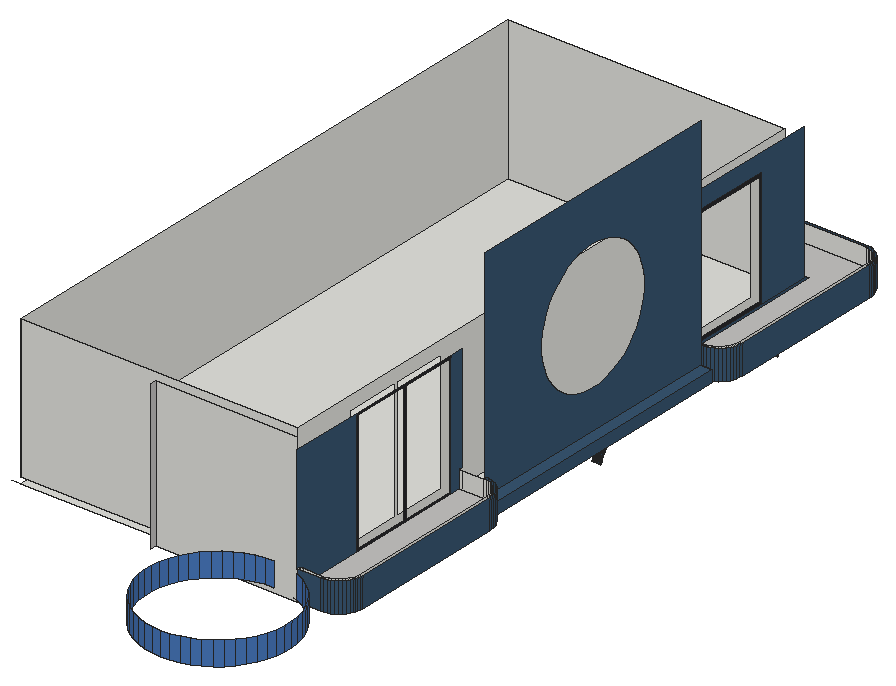
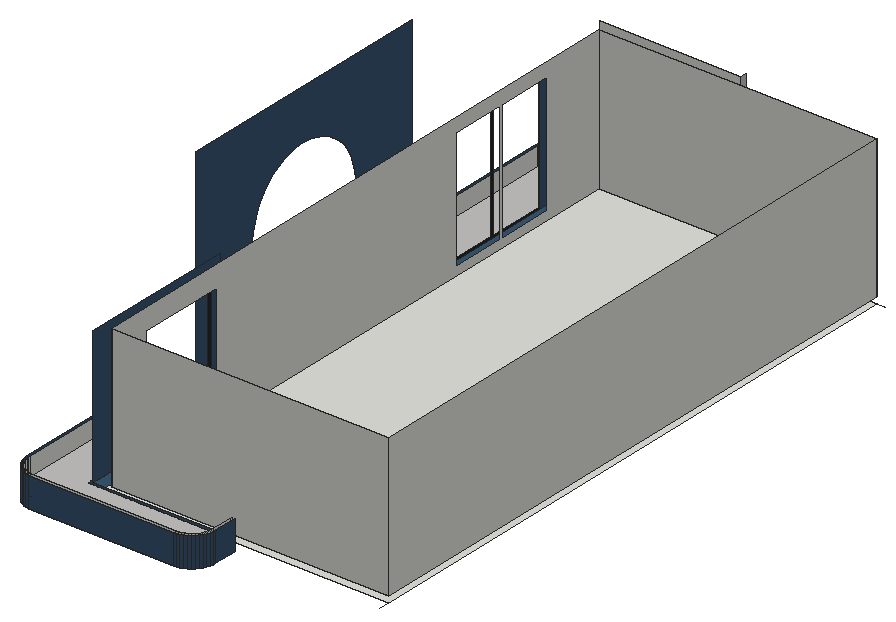
# SketchUp Ruby script. Lengths in inches.
U = 1.inch
M = Sketchup.active_model
def pt(a) = Geom::Point3d.new(a.map { |v| v * U })
def face(e, loops, mat)
  f = e.add_face(loops[0].map { |a| pt(a) })
  loops[1..].each { |l| e.add_face(l.map { |a| pt(a) }).erase! }
  f.material = f.back_material = mat if mat
  f
end
# faces: each face lists its corners as indices into pts; further lists are holes
def faces(e, pts, list, mat = nil) = list.each { |f| face(e, (f[0].is_a?(Array) ? f : [f]).map { |l| l.map { |i| pts[i] } }, mat) }
# xy, xz, yz: faces in a plane at the given z, y or x. An outline is a flat list of corners, or four numbers for a rectangle; further outlines are holes
def ring(l) = l.size == 4 ? [[l[0], l[1]], [l[2], l[1]], [l[2], l[3]], [l[0], l[3]]] : l.each_slice(2).to_a
def flat(e, list, mat, &to3) = list.each { |f| face(e, (f[0].is_a?(Array) ? f : [f]).map { |l| ring(l).map { |u, v| to3.(u, v) } }, mat) }
def xy(e, z, list, mat = nil) = flat(e, list, mat) { |x, y| [x, y, z] }
def xz(e, y, list, mat = nil) = flat(e, list, mat) { |x, z| [x, y, z] }
def yz(e, x, list, mat = nil) = flat(e, list, mat) { |y, z| [x, y, z] }
def lines(e, pts, list) = list.each { |a, b| e.add_line(pt(pts[a]), pt(pts[b])) }
# prism: a flat outline (further loops are holes) pulled along v
def prism(e, loops, v, mat = nil)
  f = face(e, loops, mat); d = Geom::Vector3d.new(v.map { |x| x * U })
  f.pushpull(f.normal.samedirection?(d) ? d.length : -d.length)
end
def box(e, o, s, mat = nil) = prism(e, [[o, [o[0] + s[0], o[1], o[2]], [o[0] + s[0], o[1] + s[1], o[2]], [o[0], o[1] + s[1], o[2]]]], [0, 0, s[2]], mat)
def at(x, y, z, deg = 0) = Geom::Transformation.translation(pt([x, y, z])) * Geom::Transformation.rotation(ORIGIN, Z_AXIS, deg.degrees)
def axes(o, x, y, z) = Geom::Transformation.new([*x, 0, *y, 0, *z, 0, *pt(o).to_a, 1])
def part(name) = M.definitions.add(name)
# library, detail: a bought-in or finely detailed component or shape, given as its bounding box
def library(name, o, s) = part(name).tap { |d| box(d.entities, o, s) }
def detail(e, o, s) = box(e.add_group.entities, o, s)
def put(e, d, t, mat = nil) = e.add_instance(d, t).tap { |i| i.material = mat if mat }
def group(e, t, mat = nil) = e.add_group.tap { |g| g.transformation = t; g.material = mat if mat }.entities
root = M.entities
M.materials.add("Carpet_01_1K").color = [196, 195, 193]
M.materials.add("Carpet_04_1K").color = [56, 85, 112]
M.materials.add("Carpet_04_1K1").color = [43, 65, 85]
M.materials.add("Glass_Mirror_01").color = [71, 118, 185]
M.materials.add("ThomThom - Buttons2").color = [40, 40, 43]
xy(root,276,[[321.57,573.58,330.57,734.38]],"Carpet_04_1K1")
xy(root,294,[[321.57,167.5625,330.57,238.58],[321.57,246.62,330.57,321.66],[321.57,329.7,330.57,404.74]])
xy(root,300,[[321.57,155.5,330.57,798.7],[39.57,167.5625,321.57,786.64]])
xy(root,300,[[330.57,155.5,330.57,798.7,186.57,798.7,186.57,822.7,186.78,825.83,187.39,828.91,188.4,831.89,189.79,834.7,191.53,837.3125,193.6,839.67,195.96,841.74,198.57,843.49,201.39,844.875,204.36,845.88,207.44,846.5,210.57,846.7,357.88,846.7,360.79,846.12,363.76,845.11,366.57,843.73,369.19,841.98,371.55,839.91,373.62,837.55,375.36,834.94,376.75,832.125,377.76,829.15,378.37,826.07,378.57,822.94,378.57,661.9,378.37,658.77,377.76,655.6875,376.75,652.72,375.36,649.9,373.62,647.29,371.55,644.93,369.19,642.86,366.57,641.12,363.76,639.73,360.79,638.72,357.71,638.11,354.57,637.9,366.57,637.9,366.57,364.54,354.57,364.54,357.71,364.34,360.79,363.72,363.76,362.71,366.57,361.33,369.19,359.58,371.55,357.51,373.62,355.15,375.36,352.54,376.75,349.73,377.76,346.75,378.37,343.67,378.57,340.54,378.57,179.5,378.37,176.37,377.76,173.29,377.18,171.58,376.75,170.32,375.36,167.5,373.62,164.89,371.55,162.53,369.19,160.46,366.57,158.72,363.76,157.33,360.79,156.32,357.71,155.71,354.57,155.5]],"Carpet_04_1K")
xy(root,306,[[39.57,167.5625,321.57,786.64]])
xy(root,312,[[330.57,158.5,354.57,158.5,357.32,158.68,360.01,159.22,362.61,160.1,365.07,161.3125,367.36,162.84,369.42,164.65,371.24,166.72,372.76,169,373.98,171.46,374.86,174.07,375.4,176.76,375.57,179.5,375.57,340.54,375.4,343.28,374.86,345.98,373.98,348.58,372.76,351.04,371.24,353.32,369.42,355.39,367.36,357.2,365.07,358.73,362.61,359.94,360.01,360.83,357.32,361.36,354.57,361.54,330.57,361.54],[333.57,640.9,354.57,640.9,357.32,641.08,360.01,641.62,362.61,642.5,365.07,643.71,367.36,645.24,369.42,647.05,371.24,649.12,372.76,651.4,373.98,653.86,374.86,656.47,375.4,659.16,375.57,661.9,375.57,822.84,375.39,825.68,374.85,828.375,373.97,830.97,372.76,833.4375,371.23,835.72,369.42,837.79,367.36,839.6,365.07,841.12,362.61,842.34,360.01,843.22,357.59,843.7,210.57,843.7,207.83,843.52,205.14,842.99,202.54,842.1,200.07,840.89,197.79,839.36,195.73,837.55,193.91,835.48,192.39,833.2,191.17,830.74,190.29,828.14,189.75,825.44,189.57,822.7,189.57,801.7,333.57,801.7]],"Carpet_01_1K")
xy(root,312,[[354.57,364.54,366.57,637.9]],"Carpet_04_1K")
xy(root,312,[[330.57,640.9,333.57,640.9,333.57,801.7,189.57,801.7,189.57,798.7,330.57,798.7]],"Carpet_04_1K1")
xz(root,155.5,[[186.57,300,330.57,450]])
xz(root,155.5,[[330.57,300,354.57,330]],"Carpet_04_1K")
xz(root,158.5,[[330.57,312,333.57,330],[333.57,312,354.57,330]])
xz(root,167.5625,[[39.57,306,321.57,450]])
xz(root,361.54,[[330.57,312,333.57,330],[333.57,312,354.57,330]])
xz(root,364.54,[[354.57,300,366.57,312],[354.57,312,354.58,330]])
xz(root,637.9,[[354.57,300,366.57,312]])
xz(root,640.9,[[330.57,312,333.57,330],[333.57,312,354.57,330]])
xz(root,786.64,[[39.57,306,321.57,450]])
xz(root,843.7,[[210.57,312,357.59,330]])
xz(root,846.7,[[210.57,300,357.88,330]],"Carpet_04_1K")
yz(root,39.57,[[167.5625,306,786.64,450]])
yz(root,186.57,[[149.51,300,155.5,450]],"Carpet_01_1K")
yz(root,186.57,[[798.7,300,822.7,330]],"Carpet_04_1K")
yz(root,189.57,[[798.7,312,801.7,330],[801.7,312,822.7,330]])
yz(root,236.92,[[77.22,306,86.26,330]],"Glass_Mirror_01")
yz(root,321.57,[[[167.5625,306,786.64,450],[652.9,315,742.9,429],[233.15,314,291.15,436],[293.15,314,349.15,436]]])
yz(root,330.57,[[158.5,312,231.15,312,231.15,438,155.5,438,155.5,330,158.5,330],[351.15,312,361.54,312,361.54,330,364.54,330,364.54,438,351.15,438],[640.9,312,649.9,312,649.9,432,745.9,432,745.9,312,798.7,312,798.7,450,637.9,450,637.9,330,640.9,330]],"Carpet_04_1K")
yz(root,330.57,[[[231.15,312,351.15,438],[233.15,314,233.15,436,349.15,436,349.15,314,293.15,314,293.15,436,291.15,436,291.15,314]],[[649.9,312,745.9,432],[652.9,315,742.9,429]]],"ThomThom - Buttons2")
yz(root,354.57,[[[364.54,312,637.9,534],[501.17,351,492.9,351.53,484.76,353.09,476.875,355.65,469.38,359.1875,462.39,363.64,456,368.92,450.33,374.97,445.47,381.68,441.48,388.95,438.44,396.65,436.38,404.68,435.35,412.91,435.35,421.2,436.4,429.42,438.47,437.44,441.52,445.15,445.52,452.41,450.4,459.11,456.08,465.15,462.47,470.43,469.47,474.86,476.97,478.38,484.86,480.9375,493,482.49,501.22,483,501.27,483,509.54,482.47,517.68,480.91,525.57,478.35,533.0625,474.8125,540.06,470.36,546.4375,465.08,552.11,459.03,556.97,452.32,560.96,445.05,564.01,437.35,566.0625,429.32,567.09,421.09,567.09,412.8,566.04,404.58,563.97,396.56,560.92,388.85,556.92,381.59,552.04,374.89,546.36,368.85,539.97,363.57,532.97,359.14,525.47,355.62,517.58,353.0625,509.44,351.51]]],"Carpet_04_1K")
yz(root,366.57,[[364.54,300,637.9,312]],"Carpet_04_1K")
yz(root,375.57,[[179.5,312,340.54,330],[661.9,312,822.84,330]])
yz(root,378.57,[[179.5,300,340.54,330],[661.9,300,822.94,330]],"Carpet_04_1K")
yz(root,380.64,[[77.22,306,86.26,330]],"Glass_Mirror_01")
p = [[330.57,541.82,255.75],[330.57,541.67,255.01],[321.57,541.67,255.01],[321.57,541.82,255.75],[330.57,766.29,255.01],[330.57,766.14,255.75],
  [321.57,766.14,255.75],[321.57,766.29,255.01],[330.57,541.99,256.5],[321.57,541.99,256.5],[330.57,765.97,256.5],[321.57,765.97,256.5],
  [330.57,542.2,257.24],[321.57,542.2,257.24],[330.57,765.77,257.24],[321.57,765.77,257.24],[330.57,542.43,257.97],[321.57,542.43,257.97],
  [330.57,765.53,257.97],[321.57,765.53,257.97],[330.57,542.7,258.7],[321.57,542.7,258.7],[330.57,765.26,258.7],[321.57,765.26,258.7],
  [330.57,542.99,259.42],[321.57,542.99,259.42],[330.57,764.97,259.42],[321.57,764.97,259.42],[330.57,543.32,260.13],[321.57,543.32,260.13],
  [330.57,764.64,260.13],[321.57,764.64,260.13],[330.57,543.68,260.83],[321.57,543.68,260.83],[330.57,764.28,260.83],[321.57,764.28,260.83],
  [330.57,544.07,261.53],[321.57,544.07,261.53],[330.57,763.9,261.53],[321.57,763.9,261.53],[330.57,544.48,262.22],[321.57,544.48,262.22],
  [330.57,763.48,262.22],[321.57,763.48,262.22],[330.57,544.93,262.9],[321.57,544.93,262.9],[330.57,763.04,262.9],[321.57,763.04,262.9],
  [330.57,545.4,263.5625],[321.57,545.4,263.5625],[330.57,762.5625,263.5625],[321.57,762.5625,263.5625],[330.57,545.9,264.22],[321.57,545.9,264.22],
  [330.57,762.0625,264.22],[321.57,762.0625,264.22],[330.57,546.43,264.86],[321.57,546.43,264.86],[330.57,761.53,264.86],[321.57,761.53,264.86],
  [330.57,546.98,265.49],[321.57,546.98,265.49],[330.57,760.98,265.49],[321.57,760.98,265.49],[330.57,547.5625,266.11],[321.57,547.5625,266.11],
  [330.57,760.4,266.11],[321.57,760.4,266.11],[330.57,548.17,266.71],[321.57,548.17,266.71],[330.57,759.79,266.71],[321.57,759.79,266.71],
  [330.57,548.8,267.3],[321.57,548.8,267.3],[330.57,759.16,267.3],[321.57,759.16,267.3],[330.57,549.46,267.87],[321.57,549.46,267.87],
  [330.57,758.5,267.87],[321.57,758.5,267.87],[330.57,550.14,268.43],[321.57,550.14,268.43],[330.57,757.82,268.43],[321.57,757.82,268.43],
  [330.57,550.84,268.97],[321.57,550.84,268.97],[330.57,757.12,268.97],[321.57,757.12,268.97],[330.57,551.57,269.5],[321.57,551.57,269.5],
  [330.57,756.4,269.5],[321.57,756.4,269.5],[330.57,552.3125,270],[321.57,552.3125,270],[330.57,755.65,270],[321.57,755.65,270],
  [330.57,553.08,270.49],[321.57,553.08,270.49],[330.57,754.88,270.49],[321.57,754.88,270.49],[330.57,553.87,270.96],[321.57,553.87,270.96],
  [330.57,754.09,270.96],[321.57,754.09,270.96],[330.57,554.68,271.42],[321.57,554.68,271.42],[330.57,753.28,271.42],[321.57,753.28,271.42],
  [330.57,555.5,271.85],[321.57,555.5,271.85],[330.57,752.46,271.85],[321.57,752.46,271.85],[330.57,556.35,272.26],[321.57,556.35,272.26],
  [330.57,751.61,272.26],[321.57,751.61,272.26],[330.57,557.21,272.66],[321.57,557.21,272.66],[330.57,750.75,272.66],[321.57,750.75,272.66],
  [330.57,558.09,273.03],[321.57,558.09,273.03],[330.57,749.875,273.03],[321.57,749.875,273.03],[330.57,558.98,273.38],[321.57,558.98,273.38],
  [330.57,748.98,273.38],[321.57,748.98,273.38],[330.57,559.89,273.72],[321.57,559.89,273.72],[330.57,748.07,273.72],[321.57,748.07,273.72],
  [330.57,560.81,274.03],[321.57,560.81,274.03],[330.57,747.15,274.03],[321.57,747.15,274.03],[330.57,561.74,274.31],[321.57,561.74,274.31],
  [330.57,746.22,274.31],[321.57,746.22,274.31],[330.57,562.6875,274.58],[321.57,562.6875,274.58],[330.57,745.27,274.58],[321.57,745.27,274.58],
  [330.57,563.64,274.83],[321.57,563.64,274.83],[330.57,744.32,274.83],[321.57,744.32,274.83],[330.57,564.61,275.05],[321.57,564.61,275.05],
  [330.57,743.35,275.05],[321.57,743.35,275.05],[330.57,565.58,275.25],[321.57,565.58,275.25],[330.57,742.38,275.25],[321.57,742.38,275.25],
  [330.57,566.57,275.42],[321.57,566.57,275.42],[330.57,741.4,275.42],[321.57,741.4,275.42],[330.57,567.55,275.57],[321.57,567.55,275.57],
  [330.57,740.41,275.57],[321.57,740.41,275.57],[330.57,568.55,275.7],[321.57,568.55,275.7],[330.57,739.41,275.7],[321.57,739.41,275.7],
  [330.57,569.55,275.8125],[321.57,569.55,275.8125],[330.57,738.41,275.8125],[321.57,738.41,275.8125],[330.57,570.55,275.89],[321.57,570.55,275.89],
  [330.57,737.41,275.89],[321.57,737.41,275.89],[330.57,571.5625,275.95],[321.57,571.5625,275.95],[330.57,736.4,275.95],[321.57,736.4,275.95],
  [330.57,572.57,275.99],[321.57,572.57,275.99],[330.57,573.58,276],[321.57,573.58,276],[330.57,735.39,275.99],[330.57,734.38,276],
  [321.57,734.38,276],[321.57,735.39,275.99],[357.71,155.71,300],[357.71,155.71,330],[354.57,155.5,330],[354.57,155.5,300],
  [360.79,156.32,300],[360.79,156.32,330],[363.76,157.33,300],[363.76,157.33,330],[366.57,158.72,300],[366.57,158.72,330],
  [369.19,160.46,300],[369.19,160.46,330],[371.55,162.53,300],[371.55,162.53,330],[373.62,164.89,300],[373.62,164.89,330],
  [375.36,167.5,300],[375.36,167.5,330],[376.75,170.32,300],[376.75,170.32,330],[377.18,171.58,300],[377.18,171.58,330],
  [377.76,173.29,300],[377.76,173.29,330],[378.37,176.37,300],[378.37,176.37,330],[378.57,179.5,300],[378.57,179.5,330],
  [378.37,343.67,300],[378.37,343.67,330],[378.57,340.54,330],[378.57,340.54,300],[377.76,346.75,300],[377.76,346.75,330],
  [376.75,349.73,300],[376.75,349.73,330],[375.36,352.54,300],[375.36,352.54,330],[373.62,355.15,300],[373.62,355.15,330],
  [371.55,357.51,300],[371.55,357.51,330],[369.19,359.58,300],[369.19,359.58,330],[366.57,361.33,300],[366.57,361.33,330],
  [363.76,362.71,300],[363.76,362.71,330],[360.79,363.72,300],[360.79,363.72,330],[357.71,364.34,300],[357.71,364.34,330],
  [354.57,364.54,312],[354.58,364.54,312],[354.58,364.54,330],[354.57,364.54,300],[357.71,638.11,300],[357.71,638.11,330],
  [354.57,637.9,330],[354.57,637.9,312],[354.57,637.9,300],[360.79,638.72,300],[360.79,638.72,330],[363.76,639.73,300],
  [363.76,639.73,330],[366.57,641.12,300],[366.57,641.12,330],[369.19,642.86,300],[369.19,642.86,330],[371.55,644.93,300],
  [371.55,644.93,330],[373.62,647.29,300],[373.62,647.29,330],[375.36,649.9,300],[375.36,649.9,330],[376.75,652.72,300],
  [376.75,652.72,330],[377.76,655.6875,300],[377.76,655.6875,330],[378.37,658.77,300],[378.37,658.77,330],[378.57,661.9,300],
  [378.57,661.9,330],[186.57,822.7,300],[186.57,822.7,330],[186.78,825.83,330],[186.78,825.83,300],[378.37,826.07,300],
  [378.37,826.07,330],[378.57,822.94,330],[378.57,822.94,300],[187.39,828.91,330],[187.39,828.91,300],[377.76,829.15,300],
  [377.76,829.15,330],[188.4,831.89,330],[188.4,831.89,300],[376.75,832.125,300],[376.75,832.125,330],[189.79,834.7,330],
  [189.79,834.7,300],[375.36,834.94,300],[375.36,834.94,330],[191.53,837.3125,330],[191.53,837.3125,300],[373.62,837.55,300],
  [373.62,837.55,330],[193.6,839.67,330],[193.6,839.67,300],[371.55,839.91,300],[371.55,839.91,330],[195.96,841.74,330],
  [195.96,841.74,300],[369.19,841.98,300],[369.19,841.98,330],[198.57,843.49,330],[198.57,843.49,300],[366.57,843.73,300],
  [366.57,843.73,330],[201.39,844.875,330],[201.39,844.875,300],[363.76,845.11,300],[363.76,845.11,330],[204.36,845.88,330],
  [204.36,845.88,300],[360.79,846.12,300],[360.79,846.12,330],[207.44,846.5,330],[207.44,846.5,300],[357.88,846.7,312],
  [357.88,846.7,330],[357.88,846.7,300],[210.57,846.7,330],[210.57,846.7,300],[308.78,9.74,306],[308.78,9.74,330],
  [299.76,10.3,330],[299.76,10.3,306],[317.8,10.3,306],[317.8,10.3,330],[290.875,12,330],[290.875,12,306],
  [326.6875,12,306],[326.6875,12,330],[282.28,14.79,330],[282.28,14.79,306],[335.29,14.79,306],[335.29,14.79,330],
  [274.09,18.64,330],[274.09,18.64,306],[343.47,18.64,306],[343.47,18.64,330],[266.46,23.49,330],[266.46,23.49,306],
  [351.1,23.49,306],[351.1,23.49,330],[259.49,29.25,330],[259.49,29.25,306],[358.07,29.25,306],[358.07,29.25,330],
  [253.3,35.84,330],[253.3,35.84,306],[364.26,35.84,306],[364.26,35.84,330],[247.99,43.16,330],[247.99,43.16,306],
  [369.57,43.16,306],[369.57,43.16,330],[243.63,51.08,330],[243.63,51.08,306],[373.93,51.08,306],[373.93,51.08,330],
  [240.3,59.49,330],[240.3,59.49,306],[377.26,59.49,306],[377.26,59.49,330],[238.06,68.25,330],[238.06,68.25,306],
  [379.51,68.25,306],[379.51,68.25,330],[236.92,77.22,330],[236.92,77.22,306],[380.64,77.22,306],[380.64,77.22,330],
  [236.92,86.26,306],[236.92,86.26,330],[238.06,95.23,330],[238.06,95.23,306],[379.51,95.23,306],[379.51,95.23,330],
  [380.64,86.26,330],[380.64,86.26,306],[240.3,103.99,330],[240.3,103.99,306],[377.26,103.99,306],[377.26,103.99,330],
  [243.63,112.39,330],[243.63,112.39,306],[373.93,112.39,306],[373.93,112.39,330],[247.99,120.32,330],[247.99,120.32,306],
  [369.57,120.32,306],[369.57,120.32,330],[253.3,127.63,330],[253.3,127.63,306],[364.26,127.63,306],[364.26,127.63,330],
  [259.49,134.22,330],[259.49,134.22,306],[358.07,134.22,306],[358.07,134.22,330],[266.46,139.99,330],[266.46,139.99,306],
  [351.1,139.99,306],[351.1,139.99,330],[274.09,144.83,330],[274.09,144.83,306],[343.47,144.83,306],[343.47,144.83,330],
  [282.28,148.68,330],[282.28,148.68,306],[335.29,148.68,306],[335.29,148.68,330],[290.875,151.48,330],[290.875,151.48,306],
  [299.76,153.17,330],[299.76,153.17,306],[308.78,153.74,330],[308.78,153.74,306],[357.32,158.68,312],[354.57,158.5,312],
  [354.57,158.5,330],[357.32,158.68,330],[360.01,159.22,312],[360.01,159.22,330],[362.61,160.1,312],[362.61,160.1,330],
  [365.07,161.3125,312],[365.07,161.3125,330],[367.36,162.84,312],[367.36,162.84,330],[369.42,164.65,312],[369.42,164.65,330],
  [371.24,166.72,312],[371.24,166.72,330],[372.76,169,312],[372.76,169,330],[373.98,171.46,312],[373.98,171.46,330],
  [374.86,174.07,312],[374.86,174.07,330],[375.4,176.76,312],[375.4,176.76,330],[375.57,179.5,312],[375.57,179.5,330],
  [375.4,343.28,312],[375.57,340.54,312],[375.57,340.54,330],[375.4,343.28,330],[374.86,345.98,312],[374.86,345.98,330],
  [373.98,348.58,312],[373.98,348.58,330],[372.76,351.04,312],[372.76,351.04,330],[371.24,353.32,312],[371.24,353.32,330],
  [369.42,355.39,312],[369.42,355.39,330],[367.36,357.2,312],[367.36,357.2,330],[365.07,358.73,312],[365.07,358.73,330],
  [362.61,359.94,312],[362.61,359.94,330],[360.01,360.83,312],[360.01,360.83,330],[357.32,361.36,312],[357.32,361.36,330],
  [354.57,361.54,312],[354.57,361.54,330],[357.32,641.08,312],[354.57,640.9,312],[354.57,640.9,330],[357.32,641.08,330],
  [360.01,641.62,312],[360.01,641.62,330],[362.61,642.5,312],[362.61,642.5,330],[365.07,643.71,312],[365.07,643.71,330],
  [367.36,645.24,312],[367.36,645.24,330],[369.42,647.05,312],[369.42,647.05,330],[371.24,649.12,312],[371.24,649.12,330],
  [372.76,651.4,312],[372.76,651.4,330],[373.98,653.86,312],[373.98,653.86,330],[374.86,656.47,312],[374.86,656.47,330],
  [375.4,659.16,312],[375.4,659.16,330],[375.57,661.9,312],[375.57,661.9,330],[189.57,822.7,312],[189.75,825.44,312],
  [189.75,825.44,330],[189.57,822.7,330],[375.39,825.68,312],[375.57,822.84,312],[375.57,822.84,330],[375.39,825.68,330],
  [190.29,828.14,312],[190.29,828.14,330],[374.85,828.375,312],[374.85,828.375,330],[191.17,830.74,312],[191.17,830.74,330],
  [373.97,830.97,312],[373.97,830.97,330],[192.39,833.2,312],[192.39,833.2,330],[372.76,833.4375,312],[372.76,833.4375,330],
  [193.91,835.48,312],[193.91,835.48,330],[371.23,835.72,312],[371.23,835.72,330],[195.73,837.55,312],[195.73,837.55,330],
  [369.42,837.79,312],[369.42,837.79,330],[197.79,839.36,312],[197.79,839.36,330],[367.36,839.6,312],[367.36,839.6,330],
  [200.07,840.89,312],[200.07,840.89,330],[365.07,841.12,312],[365.07,841.12,330],[202.54,842.1,312],[202.54,842.1,330],
  [362.61,842.34,312],[362.61,842.34,330],[205.14,842.99,312],[205.14,842.99,330],[360.01,843.22,312],[360.01,843.22,330],
  [207.83,843.52,312],[207.83,843.52,330],[357.59,843.7,312],[357.59,843.7,330],[210.57,843.7,312],[210.57,843.7,330],
  [39.57,167.5625,300],[30.57,167.5625,300],[39.57,786.64,300],[39.57,798.7,300],[357.71,846.74,312],[354.57,846.94,312],
  [330.57,150.21,306]]
faces(root,p,[[0,1,2,3],[4,5,6,7],[8,0,3,9],[5,10,11,6],[12,8,9,13],[10,14,15,11],[16,12,13,17],[14,18,19,15],
  [20,16,17,21],[18,22,23,19],[24,20,21,25],[22,26,27,23],[28,24,25,29],[26,30,31,27],[32,28,29,33],[30,34,35,31],
  [36,32,33,37],[34,38,39,35],[40,36,37,41],[38,42,43,39],[44,40,41,45],[42,46,47,43],[48,44,45,49],[46,50,51,47],
  [52,48,49,53],[50,54,55,51],[56,52,53,57],[54,58,59,55],[60,56,57,61],[58,62,63,59],[64,60,61,65],[62,66,67,63],
  [68,64,65,69],[66,70,71,67],[72,68,69,73],[70,74,75,71],[76,72,73,77],[74,78,79,75],[80,76,77,81],[78,82,83,79],
  [84,80,81,85],[82,86,87,83],[88,84,85,89],[86,90,91,87],[92,88,89,93],[90,94,95,91],[96,92,93,97],[94,98,99,95],
  [100,96,97,101],[98,102,103,99],[104,100,101,105],[102,106,107,103],[108,104,105,109],[106,110,111,107],[112,108,109,113],[110,114,115,111],
  [116,112,113,117],[114,118,119,115],[120,116,117,121],[118,122,123,119],[124,120,121,125],[122,126,127,123],[128,124,125,129],[126,130,131,127],
  [132,128,129,133],[130,134,135,131],[136,132,133,137],[134,138,139,135],[140,136,137,141],[138,142,143,139],[144,140,141,145],[142,146,147,143],
  [148,144,145,149],[146,150,151,147],[152,148,149,153],[150,154,155,151],[156,152,153,157],[154,158,159,155],[160,156,157,161],[158,162,163,159],
  [164,160,161,165],[162,166,167,163],[168,164,165,169],[166,170,171,167],[172,168,169,173],[170,174,175,171],[176,172,173,177],[174,178,179,175],
  [180,176,177,181],[182,180,181,183],[184,185,186,187],[178,184,187,179]],"Carpet_04_1K1")
faces(root,p,[[188,189,190,191],[192,193,189,188],[194,195,193,192],[196,197,195,194],[198,199,197,196],[200,201,199,198],[202,203,201,200],[204,205,203,202],
  [206,207,205,204],[208,209,207,206],[210,211,209,208],[212,213,211,210],[214,215,213,212],[216,217,218,219],[220,221,217,216],[222,223,221,220],
  [224,225,223,222],[226,227,225,224],[228,229,227,226],[230,231,229,228],[232,233,231,230],[234,235,233,232],[236,237,235,234],[238,239,237,236],
  [240,241,242,239,238,243],[244,245,246,247,248],[249,250,245,244],[251,252,250,249],[253,254,252,251],[255,256,254,253],[257,258,256,255],[259,260,258,257],
  [261,262,260,259],[263,264,262,261],[265,266,264,263],[267,268,266,265],[269,270,268,267],[271,272,273,274],[275,276,277,278],[274,273,279,280],
  [281,282,276,275],[280,279,283,284],[285,286,282,281],[284,283,287,288],[289,290,286,285],[288,287,291,292],[293,294,290,289],[292,291,295,296],
  [297,298,294,293],[296,295,299,300],[301,302,298,297],[300,299,303,304],[305,306,302,301],[304,303,307,308],[309,310,306,305],[308,307,311,312],
  [313,314,310,309],[312,311,315,316],[317,318,314,313,319],[316,315,320,321]],"Carpet_04_1K")
faces(root,p,[[322,323,324,325],[326,327,323,322],[325,324,328,329],[330,331,327,326],[329,328,332,333],[334,335,331,330],[333,332,336,337],[338,339,335,334],
  [337,336,340,341],[342,343,339,338],[341,340,344,345],[346,347,343,342],[345,344,348,349],[350,351,347,346],[349,348,352,353],[354,355,351,350],
  [353,352,356,357],[358,359,355,354],[357,356,360,361],[362,363,359,358],[361,360,364,365],[366,367,363,362],[365,364,368,369],[370,371,367,366],
  [372,373,374,375],[376,377,378,379],[375,374,380,381],[382,383,377,376],[381,380,384,385],[386,387,383,382],[385,384,388,389],[390,391,387,386],
  [389,388,392,393],[394,395,391,390],[393,392,396,397],[398,399,395,394],[397,396,400,401],[402,403,399,398],[401,400,404,405],[406,407,403,402],
  [405,404,408,409],[410,411,407,406],[409,408,412,413],[413,412,414,415],[415,414,416,417]],"Glass_Mirror_01")
faces(root,p,[[418,419,420,421],[422,418,421,423],[424,422,423,425],[426,424,425,427],[428,426,427,429],[430,428,429,431],[432,430,431,433],[434,432,433,435],
  [436,434,435,437],[438,436,437,439],[440,438,439,441],[442,440,441,443],[444,445,446,447],[448,444,447,449],[450,448,449,451],[452,450,451,453],
  [454,452,453,455],[456,454,455,457],[458,456,457,459],[460,458,459,461],[462,460,461,463],[464,462,463,465],[466,464,465,467],[468,466,467,469],
  [470,471,472,473],[474,470,473,475],[476,474,475,477],[478,476,477,479],[480,478,479,481],[482,480,481,483],[484,482,483,485],[486,484,485,487],
  [488,486,487,489],[490,488,489,491],[492,490,491,493],[494,492,493,495],[496,497,498,499],[500,501,502,503],[497,504,505,498],[506,500,503,507],
  [504,508,509,505],[510,506,507,511],[508,512,513,509],[514,510,511,515],[512,516,517,513],[518,514,515,519],[516,520,521,517],[522,518,519,523],
  [520,524,525,521],[526,522,523,527],[524,528,529,525],[530,526,527,531],[528,532,533,529],[534,530,531,535],[532,536,537,533],[538,534,535,539],
  [536,540,541,537],[542,538,539,543],[540,544,545,541]])
lines(root,p,[[546,547],[548,549],[317,550],[550,551],[410,552]])
